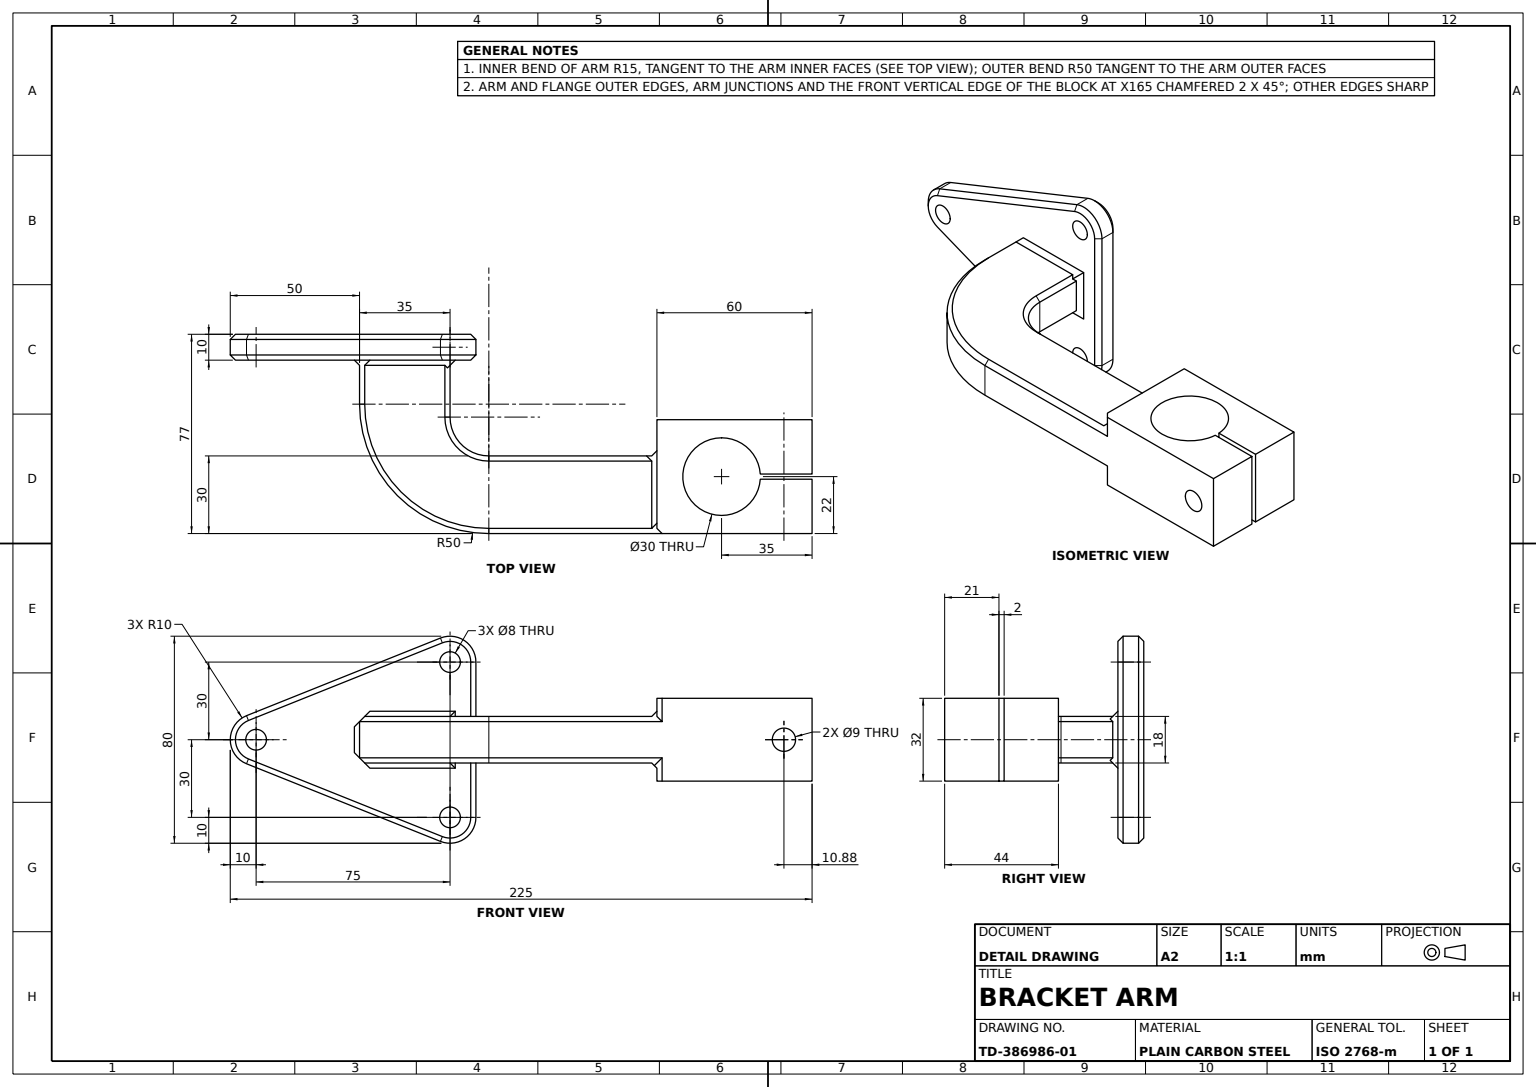
solid
v1 (-80,-9,-45)
v2 (-80,-23,-45)
e1 v1 v2 LINE
v3 (-80,-23,-65)
e2 v2 v3 LINE
v4 (-80,-9,-65)
e3 v3 v4 LINE
e4 v4 v1 LINE
face PLANE(AX(P(-80,-7,-67),D(1,0,0),D(0,0,-1))) [e1 e2 e3 e4]
v5 (-65,-25,-28)
v6 (-65,-23,-30)
e5 v5 v6 LINE
v7 (-4,-23,-30)
e6 v7 v6 LINE
v8 (-2,-25,-28)
e7 v8 v7 LINE
e8 v5 v8 LINE
face PLANE(AX(P(-65,-25,-28),D(0,0.707106781,0.707106781),D(1,0,0))) rev [e5 -e6 -e7 -e8]
v9 (-158.713907,-6.715233,-75)
v10 (-157.971125,-8.572186,-77)
e9 v9 v10 LINE
v11 (-157.971125,-23.427814,-77)
e10 v11 v10 CIRCLE(AX(P(-155,-16,-77),D(0,0,-1),D(-1,0,0)),8)
v12 (-158.713907,-25.284767,-75)
e11 v12 v11 LINE
e12 v9 v12 CIRCLE(AX(P(-155,-16,-75),D(0,0,1),D(-1,0,0)),10)
face CONE(AX(P(-155,-16,-77),D(0,0,1),D(1,0,0)),8,0.785398163) [e9 -e10 -e11 -e12]
v13 (44.619786,-16,-21)
v14 (53.619786,-16,-21)
e13 v13 v14 CIRCLE(AX(P(49.119786,-16,-21),D(0,0,1),D(1,0,0)),4.5)
v15 (44.619786,-16,0)
e14 v13 v15 LINE
v16 (53.619786,-16,0)
e15 v15 v16 CIRCLE(AX(P(49.119786,-16,0),D(0,0,1),D(1,0,0)),4.5)
e16 v14 v16 LINE
face CYL(AX(P(49.119786,-16,-60),D(0,0,1),D(1,0,0)),4.5) rev [-e13 e14 e15 -e16]
v17 (-65,-7,-2)
v18 (-2,-7,-2)
e17 v17 v18 LINE
v19 (-2,-7,-28)
e18 v18 v19 LINE
v20 (-65,-7,-28)
e19 v19 v20 LINE
v21 (-82,-7,-45)
e20 v20 v21 CIRCLE(AX(P(-65,-7,-45),D(0,-1,0),D(0,0,-1)),17)
v22 (-82,-7,-65)
e21 v21 v22 LINE
v23 (-113,-7,-65)
e22 v22 v23 LINE
v24 (-113,-7,-50)
e23 v23 v24 LINE
e24 v24 v17 CIRCLE(AX(P(-65,-7,-50),D(0,1,0),D(0,0,-1)),48)
face PLANE(AX(P(-65,-7,0),D(0,-1,0),D(0,0,-1))) rev [e17 e18 e19 e20 e21 e22 e23 e24]
v25 (2,-32,0)
v26 (0,-32,-2)
e25 v25 v26 LINE
v27 (0,-32,-44)
e26 v27 v26 LINE
v28 (60,-32,-44)
e27 v27 v28 LINE
v29 (60,-32,-23)
e28 v28 v29 LINE
v30 (39.96663,-32,-23)
e29 v30 v29 LINE
v31 (25,-32,-37)
e30 v31 v30 CIRCLE(AX(P(25,-32,-22),D(0,-1,0),D(0,0,-1)),15)
v32 (25,-32,-7)
e31 v32 v31 CIRCLE(AX(P(25,-32,-22),D(0,-1,0),D(0,0,-1)),15)
v33 (39.96663,-32,-21)
e32 v33 v32 CIRCLE(AX(P(25,-32,-22),D(0,-1,0),D(0,0,-1)),15)
v34 (60,-32,-21)
e33 v34 v33 LINE
v35 (60,-32,0)
e34 v34 v35 LINE
e35 v25 v35 LINE
face PLANE(AX(P(60,-32,-44),D(0,-1,0),D(0,0,-1))) [e25 -e26 e27 e28 -e29 -e30 -e31 -e32 -e33 e34 -e35]
v36 (-113,-25,-50)
v37 (-113,-25,-65)
e36 v36 v37 LINE
v38 (-82,-25,-65)
e37 v37 v38 LINE
v39 (-82,-25,-45)
e38 v38 v39 LINE
e39 v39 v5 CIRCLE(AX(P(-65,-25,-45),D(0,1,0),D(0,0,1)),17)
v40 (-2,-25,-2)
e40 v8 v40 LINE
v41 (-65,-25,-2)
e41 v40 v41 LINE
e42 v41 v36 CIRCLE(AX(P(-65,-25,-50),D(0,-1,0),D(0,0,1)),48)
face PLANE(AX(P(-65,-25,-30),D(0,1,0),D(0,0,1))) rev [e36 e37 e38 e39 e8 e40 e41 e42]
v42 (2,-23,0)
e43 v42 v25 LINE
v43 (60,0,0)
e44 v35 v43 LINE
v44 (2,0,0)
e45 v43 v44 LINE
v45 (2,-9,0)
e46 v44 v45 LINE
v46 (-65,-9,0)
e47 v45 v46 LINE
v47 (-65,-23,0)
e48 v47 v46 LINE
e49 v47 v42 LINE
e50 v16 v15 CIRCLE(AX(P(49.119786,-16,0),D(0,0,1),D(1,0,0)),4.5)
face PLANE(AX(P(0,0,0),D(0,0,-1),D(-1,0,0))) rev [e43 e35 e44 e45 e46 e47 -e48 e49] [-e50 -e15]
v48 (-81,-24,-64)
e51 v48 v38 LINE
e52 v3 v48 LINE
e53 v39 v2 LINE
face PLANE(AX(P(-82,-25,-30),D(0.707106781,-0.707106781,0),D(0,0,-1))) [-e38 -e51 -e52 -e2 -e53]
v49 (0,0,-2)
e54 v49 v44 LINE
v50 (0,-7,-2)
e55 v50 v49 LINE
e56 v45 v50 LINE
face PLANE(AX(P(2,0,0),D(-0.707106781,0,0.707106781),D(0,1,0))) [-e54 -e55 -e56 -e46]
v51 (-83.713907,-55.284767,-75)
e57 v12 v51 LINE
v52 (-82.971125,-53.427814,-77)
e58 v52 v11 LINE
e59 v51 v52 LINE
face PLANE(AX(P(-103.660781,-45.151951,-77),D(-0.262612866,-0.656532164,-0.707106781),D(0.928476691,-0.371390676,0))) [-e57 e11 -e58 -e59]
v53 (0,-5,-4)
e60 v53 v18 LINE
v54 (0,-5,-32)
e61 v54 v53 LINE
v55 (-2,-7,-30)
e62 v54 v55 LINE
v56 (-4,-9,-30)
e63 v56 v55 LINE
e64 v56 v19 LINE
face PLANE(AX(P(-2,-7,0),D(0.707106781,-0.707106781,0),D(0,0,-1))) rev [-e60 -e61 e62 -e63 e64 -e18]
e65 v46 v17 LINE
e66 v53 v50 LINE
face PLANE(AX(P(-65,-7,-2),D(0,-0.707106781,-0.707106781),D(1,0,0))) rev [e60 -e17 -e65 -e47 e56 -e66]
v57 (-76,14,-67)
v58 (-76,14,-77)
e67 v57 v58 LINE
v59 (-84,14,-77)
e68 v58 v59 CIRCLE(AX(P(-80,14,-77),D(0,0,-1),D(-1,0,0)),4)
v60 (-84,14,-67)
e69 v60 v59 LINE
e70 v57 v60 CIRCLE(AX(P(-80,14,-67),D(0,0,-1),D(-1,0,0)),4)
face CYL(AX(P(-80,14,-67),D(0,0,-1),D(-1,0,0)),4) rev [e67 e68 -e69 -e70]
v61 (-163,-16,-67)
v62 (-157.971125,-23.427814,-67)
e71 v61 v62 CIRCLE(AX(P(-155,-16,-67),D(0,0,1),D(-1,0,0)),8)
v63 (-165,-16,-69)
e72 v61 v63 LINE
v64 (-158.713907,-25.284767,-69)
e73 v64 v63 CIRCLE(AX(P(-155,-16,-69),D(0,0,-1),D(-1,0,0)),10)
e74 v62 v64 LINE
face CONE(AX(P(-155,-16,-69),D(0,0,-1),D(-1,0,0)),10,0.785398163) [-e71 e72 -e73 -e74]
v65 (-83.713907,-55.284767,-69)
e75 v65 v64 LINE
v66 (-82.971125,-53.427814,-67)
e76 v66 v65 LINE
e77 v62 v66 LINE
face PLANE(AX(P(-83.713907,-55.284767,-69),D(0.262612866,0.656532164,-0.707106781),D(-0.928476691,0.371390676,0))) rev [-e75 -e76 -e77 e74]
e78 v59 v58 CIRCLE(AX(P(-80,14,-77),D(0,0,-1),D(-1,0,0)),4)
e79 v60 v57 CIRCLE(AX(P(-80,14,-67),D(0,0,-1),D(-1,0,0)),4)
face CYL(AX(P(-80,14,-67),D(0,0,-1),D(-1,0,0)),4) rev [e78 -e67 -e79 e69]
v67 (60,0,-21)
e80 v67 v34 LINE
e81 v67 v43 LINE
face PLANE(AX(P(60,0,-44),D(1,0,0),D(0,0,-1))) [-e34 -e80 e81 -e44]
v68 (25,0,-37)
v69 (25,0,-7)
e82 v68 v69 CIRCLE(AX(P(25,0,-22),D(0,1,0),D(0,0,1)),15)
e83 v69 v32 LINE
e84 v68 v31 LINE
face CYL(AX(P(25,12,-22),D(0,-1,0),D(0,0,-1)),15) rev [e82 e83 e31 -e84]
v70 (-70,-46,-75)
v71 (-70,14,-75)
e85 v70 v71 LINE
v72 (-70,14,-69)
e86 v71 v72 LINE
v73 (-70,-46,-69)
e87 v72 v73 LINE
e88 v70 v73 LINE
face PLANE(AX(P(-70,14,-77),D(-1,0,0),D(0,-1,0))) rev [e85 e86 e87 -e88]
v74 (44.619786,-16,-44)
v75 (53.619786,-16,-44)
e89 v74 v75 CIRCLE(AX(P(49.119786,-16,-44),D(0,0,-1),D(-1,0,0)),4.5)
v76 (53.619786,-16,-23)
e90 v75 v76 LINE
v77 (44.619786,-16,-23)
e91 v77 v76 CIRCLE(AX(P(49.119786,-16,-23),D(0,0,-1),D(-1,0,0)),4.5)
e92 v74 v77 LINE
face CYL(AX(P(49.119786,-16,-60),D(0,0,1),D(1,0,0)),4.5) rev [e89 e90 -e91 -e92]
v78 (-151,-16,-67)
v79 (-151,-16,-77)
e93 v78 v79 LINE
v80 (-159,-16,-67)
e94 v80 v78 CIRCLE(AX(P(-155,-16,-67),D(0,0,-1),D(-1,0,0)),4)
v81 (-159,-16,-77)
e95 v80 v81 LINE
e96 v81 v79 CIRCLE(AX(P(-155,-16,-77),D(0,0,-1),D(-1,0,0)),4)
face CYL(AX(P(-155,-16,-67),D(0,0,-1),D(-1,0,0)),4) rev [-e93 -e94 e95 e96]
e97 v79 v81 CIRCLE(AX(P(-155,-16,-77),D(0,0,-1),D(-1,0,0)),4)
v82 (-76,-46,-77)
v83 (-84,-46,-77)
e98 v82 v83 CIRCLE(AX(P(-80,-46,-77),D(0,0,-1),D(-1,0,0)),4)
e99 v83 v82 CIRCLE(AX(P(-80,-46,-77),D(0,0,-1),D(-1,0,0)),4)
v84 (-82.971125,21.427814,-77)
e100 v10 v84 LINE
v85 (-72,14,-77)
e101 v84 v85 CIRCLE(AX(P(-80,14,-77),D(0,0,-1),D(-1,0,0)),8)
v86 (-72,-46,-77)
e102 v85 v86 LINE
e103 v86 v52 CIRCLE(AX(P(-80,-46,-77),D(0,0,-1),D(-1,0,0)),8)
face PLANE(AX(P(-80,14,-77),D(0,0,-1),D(-1,0,0))) [-e78 -e68] [-e96 -e97] [-e98 -e99] [e10 e100 e101 e102 e103 e58]
v87 (-84,-46,-67)
e104 v87 v83 LINE
v88 (-76,-46,-67)
e105 v88 v87 CIRCLE(AX(P(-80,-46,-67),D(0,0,-1),D(-1,0,0)),4)
e106 v88 v82 LINE
face CYL(AX(P(-80,-46,-67),D(0,0,-1),D(-1,0,0)),4) rev [e98 -e104 -e105 e106]
v89 (-1,-26,-3)
e107 v89 v42 LINE
e108 v41 v47 LINE
e109 v40 v89 LINE
face PLANE(AX(P(0,-23,0),D(0,0.707106781,-0.707106781),D(1,0,0))) rev [e107 -e49 -e108 -e41 e109]
e110 v51 v70 CIRCLE(AX(P(-80,-46,-75),D(0,0,1),D(-1,0,0)),10)
e111 v86 v70 LINE
face CONE(AX(P(-80,-46,-77),D(0,0,1),D(1,0,0)),8,0.785398163) [-e110 e59 -e103 e111]
v90 (-78,-27,-67)
e112 v90 v48 LINE
v91 (-78,-5,-67)
e113 v91 v90 LINE
v92 (-81,-8,-64)
e114 v92 v91 LINE
e115 v92 v4 LINE
face PLANE(AX(P(-78,14,-67),D(-0.707106781,0,-0.707106781),D(0,-1,0))) rev [e52 -e112 -e113 -e114 e115 -e3]
v93 (-83.713907,23.284767,-69)
v94 (-82.971125,21.427814,-67)
e116 v93 v94 LINE
v95 (-72,14,-67)
e117 v95 v94 CIRCLE(AX(P(-80,14,-67),D(0,0,1),D(-1,0,0)),8)
e118 v72 v95 LINE
e119 v93 v72 CIRCLE(AX(P(-80,14,-69),D(0,0,-1),D(-1,0,0)),10)
face CONE(AX(P(-80,14,-69),D(0,0,-1),D(-1,0,0)),10,0.785398163) [e116 -e117 -e118 -e119]
e120 v76 v77 CIRCLE(AX(P(49.119786,-16,-23),D(0,0,-1),D(-1,0,0)),4.5)
e121 v75 v74 CIRCLE(AX(P(49.119786,-16,-44),D(0,0,-1),D(-1,0,0)),4.5)
face CYL(AX(P(49.119786,-16,-60),D(0,0,1),D(1,0,0)),4.5) rev [e92 -e120 -e90 e121]
v96 (60,0,-44)
e122 v28 v96 LINE
v97 (0,0,-44)
e123 v97 v27 LINE
e124 v96 v97 LINE
face PLANE(AX(P(0,0,-44),D(0,0,-1),D(-1,0,0))) [-e122 -e27 -e123 -e124] [-e121 -e89]
v98 (-83.713907,23.284767,-75)
e125 v98 v93 LINE
e126 v71 v98 CIRCLE(AX(P(-80,14,-75),D(0,0,1),D(-1,0,0)),10)
face CYL(AX(P(-80,14,-77),D(0,0,1),D(1,0,0)),10) [e125 e119 -e86 e126]
e127 v73 v65 CIRCLE(AX(P(-80,-46,-69),D(0,0,-1),D(-1,0,0)),10)
v99 (-72,-46,-67)
e128 v99 v73 LINE
e129 v66 v99 CIRCLE(AX(P(-80,-46,-67),D(0,0,1),D(-1,0,0)),8)
face CONE(AX(P(-80,-46,-69),D(0,0,-1),D(-1,0,0)),10,0.785398163) [e76 -e127 -e128 -e129]
e130 v84 v98 LINE
e131 v98 v9 LINE
face PLANE(AX(P(-82.971125,21.427814,-77),D(-0.262612866,0.656532164,-0.707106781),D(-0.928476691,-0.371390676,0))) [-e130 -e100 -e9 -e131]
v100 (-111,-5,-67)
e132 v100 v91 LINE
e133 v23 v100 LINE
e134 v22 v92 LINE
face PLANE(AX(P(-80,-5,-67),D(0,0.707106781,0.707106781),D(-1,0,0))) [e114 -e132 -e133 -e22 e134]
v101 (-115,-9,-65)
v102 (-115,-23,-65)
e135 v101 v102 LINE
v103 (-117,-11,-67)
e136 v103 v101 LINE
v104 (-117,-21,-67)
e137 v104 v103 LINE
e138 v102 v104 LINE
face PLANE(AX(P(-115,-7,-65),D(0.707106781,0,-0.707106781),D(0,-1,0))) rev [-e135 -e136 -e137 -e138]
v105 (-115,-9,-50)
e139 v46 v105 CIRCLE(AX(P(-65,-9,-50),D(0,-1,0),D(0,0,-1)),50)
e140 v105 v24 LINE
face CONE(AX(P(-65,-9,-50),D(0,-1,0),D(0,0,-1)),50,0.785398163) [-e139 e65 -e24 -e140]
v106 (-2,-25,-30)
e141 v55 v106 LINE
v107 (0,-27,-32)
e142 v107 v54 LINE
e143 v106 v107 LINE
face PLANE(AX(P(-2,-7,-30),D(0.707106781,0,0.707106781),D(0,-1,0))) rev [-e141 -e62 -e142 -e143]
v108 (-158.713907,-6.715233,-69)
e144 v9 v108 LINE
e145 v108 v93 LINE
face PLANE(AX(P(-83.713907,23.284767,-77),D(0.371390676,-0.928476691,0),D(0.928476691,0.371390676,0))) rev [e144 e145 -e125 e131]
v109 (-115,-23,-50)
e146 v102 v109 LINE
v110 (-111,-27,-67)
e147 v110 v104 LINE
e148 v110 v37 LINE
e149 v36 v109 LINE
face PLANE(AX(P(-113,-25,-30),D(-0.707106781,-0.707106781,0),D(0,0,1))) [-e146 e138 -e147 e148 -e36 e149]
e150 v85 v71 LINE
face PLANE(AX(P(-72,14,-77),D(0.707106781,0,-0.707106781),D(0,1,0))) [e150 -e85 -e111 -e102]
face CONE(AX(P(-80,14,-77),D(0,0,1),D(1,0,0)),8,0.785398163) [-e126 -e150 -e101 e130]
e151 v105 v101 LINE
e152 v103 v100 LINE
face PLANE(AX(P(-115,-9,-67),D(-0.707106781,0.707106781,0),D(0,0,1))) [e136 -e151 e140 -e23 e133 -e152]
e153 v90 v110 LINE
e154 v99 v95 LINE
v111 (-157.971125,-8.572186,-67)
e155 v94 v111 LINE
e156 v111 v61 CIRCLE(AX(P(-155,-16,-67),D(0,0,1),D(-1,0,0)),8)
e157 v78 v80 CIRCLE(AX(P(-155,-16,-67),D(0,0,-1),D(-1,0,0)),4)
e158 v87 v88 CIRCLE(AX(P(-80,-46,-67),D(0,0,-1),D(-1,0,0)),4)
face PLANE(AX(P(-80,14,-67),D(0,0,-1),D(-1,0,0))) rev [e79 e70] [e113 e153 e147 e137 e152 e132] [e71 e77 e129 e154 e117 e155 e156] [e94 e157] [e158 e105]
e159 v105 v109 LINE
face PLANE(AX(P(-115,-7,-67),D(-1,0,0),D(0,0,1))) [-e159 e151 e135 e146]
v112 (-65,-9,-30)
e160 v112 v20 LINE
e161 v1 v112 CIRCLE(AX(P(-65,-9,-45),D(0,1,0),D(0,0,-1)),15)
e162 v1 v21 LINE
face CONE(AX(P(-65,-9,-45),D(0,1,0),D(0,0,1)),15,0.785398163) rev [-e160 -e161 e162 -e20]
e163 v108 v111 LINE
e164 v63 v108 CIRCLE(AX(P(-155,-16,-69),D(0,0,-1),D(-1,0,0)),10)
face CONE(AX(P(-155,-16,-69),D(0,0,-1),D(-1,0,0)),10,0.785398163) [-e156 -e163 -e164 -e72]
e165 v109 v47 CIRCLE(AX(P(-65,-23,-50),D(0,1,0),D(0,0,1)),50)
face CYL(AX(P(-65,-7,-50),D(0,-1,0),D(0,0,-1)),50) [e48 e139 e159 e165]
face PLANE(AX(P(-70,14,-69),D(-0.707106781,0,-0.707106781),D(0,-1,0))) rev [e118 -e154 e128 -e87]
v113 (39.96663,0,-21)
e166 v113 v33 LINE
e167 v69 v113 CIRCLE(AX(P(25,0,-22),D(0,1,0),D(0,0,1)),15)
face CYL(AX(P(25,12,-22),D(0,-1,0),D(0,0,-1)),15) rev [e166 e32 -e83 e167]
e168 v12 v64 LINE
e169 v51 v65 LINE
face PLANE(AX(P(-83.713907,-55.284767,-77),D(0.371390676,0.928476691,0),D(-0.928476691,0.371390676,0))) rev [-e168 e57 e169 e75]
face CYL(AX(P(-80,-46,-67),D(0,0,-1),D(-1,0,0)),4) rev [-e158 e104 e99 -e106]
e170 v106 v7 LINE
e171 v112 v6 LINE
e172 v112 v56 LINE
face PLANE(AX(P(-65,-7,-30),D(0,0,1),D(1,0,0))) rev [e63 e141 e170 e6 -e171 e172]
v114 (60,0,-23)
e173 v96 v114 LINE
e174 v114 v29 LINE
face PLANE(AX(P(60,0,-44),D(1,0,0),D(0,0,-1))) [e173 e174 -e28 e122]
e175 v6 v2 CIRCLE(AX(P(-65,-23,-45),D(0,-1,0),D(0,0,1)),15)
face CYL(AX(P(-65,-7,-45),D(0,-1,0),D(0,0,-1)),15) rev [e161 e171 e175 -e1]
e176 v97 v49 LINE
v115 (0,-27,-2)
e177 v26 v115 LINE
e178 v115 v107 LINE
face PLANE(AX(P(0,-32,-44),D(-1,0,0),D(0,0,1))) [e55 -e176 e123 e26 e177 e178 e142 e61 e66]
face PLANE(AX(P(-80,-9,-67),D(0.707106781,0.707106781,0),D(0,0,-1))) [-e162 -e4 -e115 -e134 -e21]
e179 v89 v115 LINE
face PLANE(AX(P(2,0,0),D(-0.707106781,0,0.707106781),D(0,1,0))) [-e177 -e25 -e43 -e107 e179]
face PLANE(AX(P(-83.713907,23.284767,-69),D(0.262612866,-0.656532164,-0.707106781),D(0.928476691,0.371390676,0))) rev [-e116 -e145 e163 -e155]
face CONE(AX(P(-65,-25,-50),D(0,1,0),D(0,0,1)),48,0.785398163) [e108 -e165 -e149 -e42]
face PLANE(AX(P(-65,-9,-30),D(0,-0.707106781,0.707106781),D(1,0,0))) rev [e160 -e19 -e64 -e172]
e180 v14 v13 CIRCLE(AX(P(49.119786,-16,-21),D(0,0,1),D(1,0,0)),4.5)
face CYL(AX(P(49.119786,-16,-60),D(0,0,1),D(1,0,0)),4.5) rev [e50 -e14 -e180 e16]
face CYL(AX(P(-155,-16,-77),D(0,0,1),D(1,0,0)),10) [e73 e164 -e144 e12 e168]
face CYL(AX(P(-80,-46,-77),D(0,0,1),D(1,0,0)),10) [-e169 e110 e88 e127]
e181 v113 v67 LINE
v116 (39.96663,0,-23)
e182 v116 v68 CIRCLE(AX(P(25,0,-22),D(0,1,0),D(0,0,1)),15)
e183 v114 v116 LINE
face PLANE(AX(P(0,0,-44),D(0,1,0),D(0,0,1))) [e176 e54 -e45 -e81 -e181 -e167 -e82 -e182 -e183 -e173 e124]
e184 v116 v30 LINE
face PLANE(AX(P(39.96663,12,-23),D(0,0,-1),D(-1,0,0))) rev [e91 e120] [e29 -e174 e183 e184]
face PLANE(AX(P(60,12,-21),D(0,0,1),D(1,0,0))) rev [e80 e33 -e166 e181] [e13 e180]
face PLANE(AX(P(-2,-25,-30),D(0.707106781,0.707106781,0),D(0,0,1))) rev [-e40 e7 -e170 e143 -e178 -e179 -e109]
face CYL(AX(P(-155,-16,-67),D(0,0,-1),D(-1,0,0)),4) rev [e97 -e95 -e157 e93]
face CYL(AX(P(25,12,-22),D(0,-1,0),D(0,0,-1)),15) rev [e84 e30 -e184 e182]
face PLANE(AX(P(-65,-25,-65),D(0,-0.707106781,0.707106781),D(-1,0,0))) [-e37 -e148 -e153 e112 e51]
face CONE(AX(P(-65,-25,-45),D(0,-1,0),D(0,0,-1)),17,0.785398163) rev [-e175 -e5 -e39 e53]
